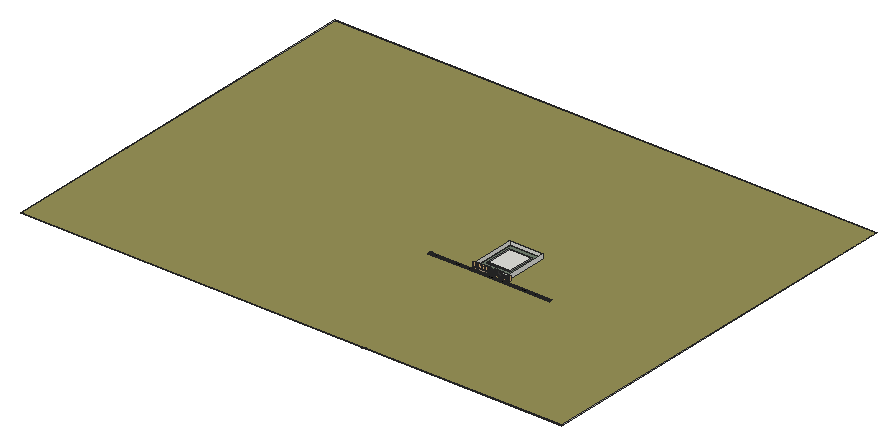
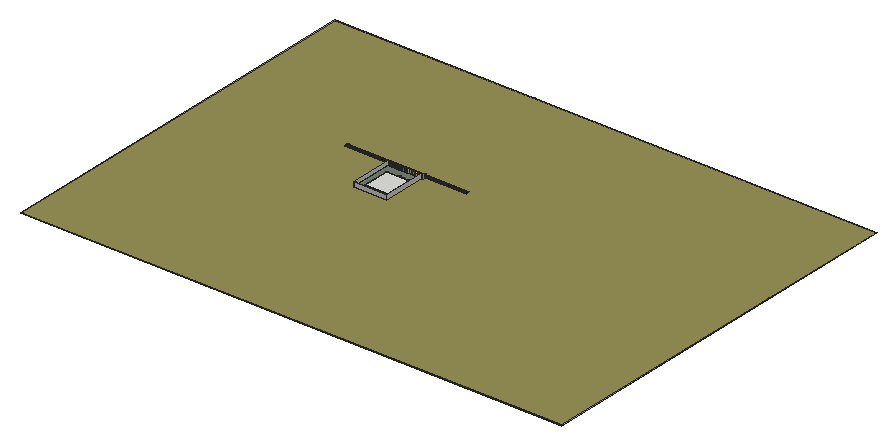
# SketchUp Ruby script. Lengths in inches.
U = 1.inch
M = Sketchup.active_model
def pt(a) = Geom::Point3d.new(a.map { |v| v * U })
def face(e, loops, mat)
  f = e.add_face(loops[0].map { |a| pt(a) })
  loops[1..].each { |l| e.add_face(l.map { |a| pt(a) }).erase! }
  f.material = f.back_material = mat if mat
  f
end
# faces: each face lists its corners as indices into pts; further lists are holes
def faces(e, pts, list, mat = nil) = list.each { |f| face(e, (f[0].is_a?(Array) ? f : [f]).map { |l| l.map { |i| pts[i] } }, mat) }
# xy, xz, yz: faces in a plane at the given z, y or x. An outline is a flat list of corners, or four numbers for a rectangle; further outlines are holes
def ring(l) = l.size == 4 ? [[l[0], l[1]], [l[2], l[1]], [l[2], l[3]], [l[0], l[3]]] : l.each_slice(2).to_a
def flat(e, list, mat, &to3) = list.each { |f| face(e, (f[0].is_a?(Array) ? f : [f]).map { |l| ring(l).map { |u, v| to3.(u, v) } }, mat) }
def xy(e, z, list, mat = nil) = flat(e, list, mat) { |x, y| [x, y, z] }
def xz(e, y, list, mat = nil) = flat(e, list, mat) { |x, z| [x, y, z] }
def yz(e, x, list, mat = nil) = flat(e, list, mat) { |y, z| [x, y, z] }
def lines(e, pts, list) = list.each { |a, b| e.add_line(pt(pts[a]), pt(pts[b])) }
# prism: a flat outline (further loops are holes) pulled along v
def prism(e, loops, v, mat = nil)
  f = face(e, loops, mat); d = Geom::Vector3d.new(v.map { |x| x * U })
  f.pushpull(f.normal.samedirection?(d) ? d.length : -d.length)
end
def box(e, o, s, mat = nil) = prism(e, [[o, [o[0] + s[0], o[1], o[2]], [o[0] + s[0], o[1] + s[1], o[2]], [o[0], o[1] + s[1], o[2]]]], [0, 0, s[2]], mat)
def at(x, y, z, deg = 0) = Geom::Transformation.translation(pt([x, y, z])) * Geom::Transformation.rotation(ORIGIN, Z_AXIS, deg.degrees)
def axes(o, x, y, z) = Geom::Transformation.new([*x, 0, *y, 0, *z, 0, *pt(o).to_a, 1])
def part(name) = M.definitions.add(name)
# library, detail: a bought-in or finely detailed component or shape, given as its bounding box
def library(name, o, s) = part(name).tap { |d| box(d.entities, o, s) }
def detail(e, o, s) = box(e.add_group.entities, o, s)
def put(e, d, t, mat = nil) = e.add_instance(d, t).tap { |i| i.material = mat if mat }
def group(e, t, mat = nil) = e.add_group.tap { |g| g.transformation = t; g.material = mat if mat }.entities
root = M.entities
M.materials.add("C07_Caramel_Shine").color = [153, 76, 0]
M.materials.add("M03_Pewter_Shine").color = [168, 168, 168]
M.materials.add("M07_Charcoal_Gleam").color = [58, 58, 58]
M.materials.add("M09_Shadow_Night").color = [0, 0, 0]
M.materials.add("Marble_01_1K").color = [230, 221, 211]
M.materials.add("Marble_06_1K").color = [165, 150, 147]
M.materials.add("Metal_06_1K").color = [238, 236, 231]
M.materials.add("Plaster_02_1K").color = [157, 140, 119]
M.materials.add("Plaster_04_1K").color = [115, 129, 112]
M.materials.add("Plaster_06_1K").color = [141, 135, 122]
M.materials.add("Plywood_01_1K").color = [125, 96, 64]
M.materials.add("Soil_04_1K").color = [152, 146, 88]
M.materials.add("Wood_Veneer_15_1K").color = [103, 69, 45]
c1 = part("Group\#38")
box(c1.entities,[0,0,0],[5,1.875,282.41],"Metal_06_1K")
c2 = library("Group\#40",[0,0,0],[80.6875,45.375,2.875])
c3 = library("Group\#39",[0,-3.0625,0],[84,3.0625,102])
c4 = part("Group\#43")
xy(c4.entities,0,[[0,-24,550.875,0]])
xy(c4.entities,12.625,[[3.37,-20.63,547.5,-3.37]],"Soil_04_1K")
xy(c4.entities,18,[[[0,-24,550.875,0],[3.37,-20.63,547.5,-3.37]]])
xz(c4.entities,-24,[[0,0,550.875,18]])
xz(c4.entities,-20.63,[[3.37,12.625,547.5,18]])
xz(c4.entities,-3.37,[[3.37,12.625,547.5,18]])
xz(c4.entities,0,[[0,0,550.875,18]])
yz(c4.entities,0,[[-24,0,0,18]])
yz(c4.entities,3.37,[[-20.63,12.625,-3.37,18]])
yz(c4.entities,547.5,[[-20.63,12.625,-3.37,18]])
yz(c4.entities,550.875,[[-24,0,0,18]])
c5 = library("Lantern 03",[-10.78,-12.92,0],[25.67,25.84,111.375])
c6 = library("Deluxe 6’ Bench",[-36.03,-11.33,0.05],[72.04,26.2,31.51])
c7 = part("Group\#46")
box(c7.entities,[0,0,0],[247.875,18.625,1])
g1 = group(root,at(8950.9375,4405.5625,0))
xy(g1,-21,[[-8950.9375,-4405.5625,5495.8125,6096.125]])
xy(g1,-18,[[-8950.9375,-4405.5625,5495.8125,6096.125]],"Soil_04_1K")
xy(g1,0,[[-38.61,-269.5,224.375,-263.5],[224.375,-269.5,250.9375,-263.5],[250.9375,-269.5,775.25,-256.625]])
xy(g1,0,[[-103.0625,-263.5,250.9375,-263.5,250.9375,-256.625,769.25,-256.625,769.25,879.875,-103.0625,879.875]],"Plaster_04_1K")
xy(g1,20.78,[[-92.4,-269.5,-59.27,-268.5]],"C07_Caramel_Shine")
xy(g1,22.41,[[-92.4,-269.5,-59.27,-268.5]],"C07_Caramel_Shine")
xy(g1,29.87,[[-92.4,-269.5,-59.27,-268.5]],"C07_Caramel_Shine")
xy(g1,31.49,[[-92.4,-269.5,-59.27,-268.5]],"C07_Caramel_Shine")
xy(g1,38.95,[[-92.4,-269.5,-59.27,-268.5]],"C07_Caramel_Shine")
xy(g1,40.58,[[-92.4,-269.5,-59.27,-268.5]],"C07_Caramel_Shine")
xy(g1,48.03,[[-92.4,-269.5,-59.27,-268.5]],"C07_Caramel_Shine")
xy(g1,49.66,[[-92.4,-269.5,-59.27,-268.5]],"C07_Caramel_Shine")
xy(g1,57.12,[[-92.4,-269.5,-59.27,-268.5]],"C07_Caramel_Shine")
xy(g1,58.74,[[-92.4,-269.5,-59.27,-268.5]],"C07_Caramel_Shine")
xy(g1,66.2,[[-92.4,-269.5,-59.27,-268.5]],"C07_Caramel_Shine")
xy(g1,67.83,[[-92.4,-269.5,-59.27,-268.5]],"C07_Caramel_Shine")
xy(g1,75.28,[[-92.4,-269.5,-59.27,-268.5]],"C07_Caramel_Shine")
xy(g1,76.91,[[-92.4,-269.5,-59.27,-268.5]],"C07_Caramel_Shine")
xy(g1,96,[[-113.0625,-263.5,-103.0625,-263.5,-103.0625,879.875,769.25,879.875,769.25,-256.625,775.25,-256.625,775.25,885.875,-113.0625,885.875]])
xy(g1,103.5,[[-113.0625,-269.5,-38.61,-263.5]])
xz(g1,-4405.5625,[[-8950.9375,-21,224.375,-18],[224.375,-21,5495.8125,-18]])
xz(g1,-269.5,[[-38.61,-18,224.375,0],[[-113.0625,0,-38.61,103.5],[-92.4,14.67,-59.27,82.01]]])
xz(g1,-269.5,[[-92.4,14.67,-59.27,20.78],[-92.4,22.41,-59.27,29.87],[-92.4,31.49,-59.27,38.95],[-92.4,40.58,-59.27,48.03],[-92.4,49.66,-59.27,57.12],
  [-92.4,58.74,-59.27,66.2],[-92.4,67.83,-59.27,75.28],[-92.4,76.91,-59.27,82.01]],"Wood_Veneer_15_1K")
xz(g1,-268.5,[[-92.4,20.78,-59.27,22.41],[-92.4,29.87,-59.27,31.49],[-92.4,38.95,-59.27,40.58],[-92.4,48.03,-59.27,49.66],[-92.4,57.12,-59.27,58.74],
  [-92.4,66.2,-59.27,67.83],[-92.4,75.28,-59.27,76.91]],"C07_Caramel_Shine")
xz(g1,-263.5,[[-103.0625,0,-38.61,103.5],[-113.0625,96,-103.0625,103.5]])
xz(g1,-256.625,[[769.25,0,775.25,96]])
xz(g1,879.875,[[-103.0625,0,769.25,96]])
xz(g1,885.875,[[-113.0625,-18,775.25,96]])
xz(g1,6096.125,[[-8950.9375,-21,5495.8125,-18]])
yz(g1,-8950.9375,[[-4405.5625,-21,-837.25,-18],[-837.25,-21,6096.125,-18]])
yz(g1,-113.0625,[[-269.5,-18,-269.5,103.5,-263.5,103.5,-263.5,96,885.875,96,885.875,-18]])
yz(g1,-103.0625,[[-263.5,0,879.875,96]])
yz(g1,-92.4,[[-269.5,20.78,-268.5,22.41],[-269.5,29.87,-268.5,31.49],[-269.5,38.95,-268.5,40.58],[-269.5,48.03,-268.5,49.66],[-269.5,57.12,-268.5,58.74],
  [-269.5,66.2,-268.5,67.83],[-269.5,75.28,-268.5,76.91]],"C07_Caramel_Shine")
yz(g1,-59.27,[[-269.5,20.78,-268.5,22.41],[-269.5,29.87,-268.5,31.49],[-269.5,38.95,-268.5,40.58],[-269.5,48.03,-268.5,49.66],[-269.5,57.12,-268.5,58.74],
  [-269.5,66.2,-268.5,67.83],[-269.5,75.28,-268.5,76.91]],"C07_Caramel_Shine")
yz(g1,-38.61,[[-269.5,0,-263.5,103.5]])
yz(g1,769.25,[[-256.625,0,879.875,96]])
yz(g1,775.25,[[-269.5,-18,885.875,-18,885.875,96,-256.625,96,-256.625,0,-269.5,0]])
yz(g1,5495.8125,[[-4405.5625,-21,6096.125,-18]])
g2 = group(g1,at(250.9375,-269.5,0))
xy(g2,0,[[-2.57,0,-2.57,8.6875,143.56,8.6875,143.56,12.875,340.42,12.875,340.42,0],[465.96,0,524.3125,12.875]])
xy(g2,24,[[-2.57,0,143.56,3.25]],"M07_Charcoal_Gleam")
xy(g2,33.26,[[183.55,0,216.43,12.875]])
xy(g2,71.1875,[[183.55,0,216.43,12.875],[340.42,0,465.96,12.875]])
xy(g2,90.75,[[-2.57,3.25,143.56,8.6875]],"Plaster_06_1K")
xy(g2,103.5,[[340.42,0,524.3125,12.875]])
xy(g2,103.5,[[143.56,0,183.55,12.875],[216.43,0,340.42,12.875]],"M07_Charcoal_Gleam")
xy(g2,107.875,[[183.55,0,216.43,12.875]])
xz(g2,0,[[465.96,0,524.3125,0,524.3125,103.5,340.42,103.5,340.42,95.1875,248.6,95.1875,248.6,71.1875,465.96,71.1875],[183.55,71.1875,216.43,107.875]])
xz(g2,0,[[-2.57,0,340.42,0,340.42,71.1875,248.6,71.1875,248.6,95.1875,340.42,95.1875,340.42,103.5,216.43,103.5,216.43,33.26,183.55,33.26,183.55,103.5,143.56,103.5,143.56,24,-2.57,24]],"M07_Charcoal_Gleam")
xz(g2,3.25,[[-2.57,24,143.56,90.75]],"Plaster_06_1K")
xz(g2,8.6875,[[-2.57,0,143.56,90.75]],"Plaster_06_1K")
xz(g2,12.875,[[465.96,0,465.96,71.1875,340.42,71.1875,340.42,103.5,518.3125,103.5,518.3125,0],[518.3125,0,524.3125,103.5]])
xz(g2,12.875,[[[143.56,0,143.56,103.5,183.55,103.5,183.55,107.875,216.43,107.875,216.43,103.5,340.42,103.5,340.42,0],[183.55,33.26,216.43,71.1875]]],"M07_Charcoal_Gleam")
yz(g2,-2.57,[[0,0,0,24,3.25,24,3.25,90.75,6,90.75,6,0],[6,0,8.6875,90.75]])
yz(g2,143.56,[[8.6875,0,8.6875,90.75,3.25,90.75,3.25,24,0,24,0,103.5,12.875,103.5,12.875,0]],"M07_Charcoal_Gleam")
yz(g2,183.55,[[0,33.26,12.875,71.1875],[0,103.5,12.875,107.875]])
yz(g2,216.43,[[0,33.26,12.875,71.1875],[0,103.5,12.875,107.875]])
yz(g2,340.42,[[0,0,12.875,71.1875]],"M07_Charcoal_Gleam")
yz(g2,465.96,[[0,0,12.875,71.1875]])
yz(g2,524.3125,[[0,0,12.875,103.5]])
put(g2,c1,axes([465.96,8.52,66.9],[0,-1,0],[0,0,1],[-1,0,0]))
put(g2,c1,axes([465.96,8.52,57.86],[0,-1,0],[0,0,1],[-1,0,0]))
put(g2,c1,axes([465.96,8.52,48.82],[0,-1,0],[0,0,1],[-1,0,0]))
put(g2,c1,axes([465.96,8.52,39.79],[0,-1,0],[0,0,1],[-1,0,0]))
put(g2,c1,axes([465.96,8.52,30.75],[0,-1,0],[0,0,1],[-1,0,0]))
put(g2,c1,axes([465.96,8.52,21.72],[0,-1,0],[0,0,1],[-1,0,0]))
put(g2,c1,axes([465.96,8.52,12.68],[0,-1,0],[0,0,1],[-1,0,0]))
put(g2,c1,axes([465.96,8.52,3.65],[0,-1,0],[0,0,1],[-1,0,0]))
put(g2,c2,axes([27.93,3.25,33.82],[1,0,0],[0,0,1],[0,-1,0]))
put(g1,c3,axes([-38.61,-266.5,0],[1.03996,0,0],[0,1,0],[0,0,0.9408]))
put(g1,c3,axes([49.66,-266.5,0],[1.03996,0,0],[0,1,0],[0,0,0.9408]))
put(g1,c3,axes([137.02,-266.5,0],[1.03996,0,0],[0,1,0],[0,0,0.9408]))
g3 = group(g1,at(-113.0625,-269.5,-18))
xy(g3,0,[[0,-24,74.46,0]])
xy(g3,12.625,[[3.37,-20.63,71.08,-3.37]],"Soil_04_1K")
xy(g3,18,[[[0,-24,74.46,0],[3.37,-20.63,71.08,-3.37]]])
xz(g3,-24,[[0,0,74.46,18]])
xz(g3,-20.63,[[3.37,12.625,71.08,18]])
xz(g3,-3.37,[[3.37,12.625,71.08,18]])
xz(g3,0,[[0,0,74.46,18]])
yz(g3,0,[[-24,0,0,18]])
yz(g3,3.37,[[-20.63,12.625,-3.37,18]])
yz(g3,71.08,[[-20.63,12.625,-3.37,18]])
yz(g3,74.46,[[-24,0,0,18]])
put(g1,c4,axes([224.375,-269.5,-18],[0.4,0,0],[0,1,0],[0,0,1]))
put(g1,c4,axes([444.72,-269.5,-18],[0.4,0,0],[0,1,0],[0,0,1]))
put(g1,c4,axes([665.07,-269.5,-18],[0.2,0,0],[0,1,0],[0,0,1]))
put(root,c5,at(8801.1,4116.48,-18))
put(root,c5,at(9769.7,4127.8,-18))
g4 = group(root,at(8912.33,4041.91,-18))
xy(g4,0,[[0,0,262.98,94.16]],"Plaster_02_1K")
yz(g4,0,[[0,0,70.16,0,70.16,13.41]],"Plaster_02_1K")
yz(g4,262.98,[[0,0,70.04,13.39,70.04,0]],"Plaster_02_1K")
p = [[262.98,94.16,18],[262.98,70.04,13.39],[262.98,0,0],[0,0,0],[0,70.16,13.41],[0,94.16,18]]
faces(g4,p,[[0,1,2,3,4,5]],"Plaster_02_1K")
g5 = group(root,at(7707.8125,3957.91,-18))
prism(g5,[[[3255.3125,84,0],[3255.3125,0,0],[1204.52,0,0],[0,0,0],[0,84,0],[1204.52,84,0]]],[0,0,1],"M09_Shadow_Night")
put(root,c6,at(8864.21,4064.76,-18),"Plywood_01_1K")
put(root,c6,at(9632.09,4062.93,-18),"Plywood_01_1K")
put(root,c6,at(9421.9,4064.97,-18),"Plywood_01_1K")
put(root,c7,at(7764.95,3998.1,-17))
put(root,c7,at(8058.52,3998.1,-17))
put(root,c7,at(8352.09,3998.1,-17))
put(root,c7,at(8645.65,3998.1,-17))
put(root,c7,at(8939.22,3998.1,-17))
put(root,c7,at(9232.79,3998.1,-17))
put(root,c7,at(9526.36,3998.1,-17))
put(root,c7,at(9819.93,3998.1,-17))
put(root,c7,at(10113.5,3998.1,-17))
put(root,c7,at(10407.07,3998.1,-17))
put(root,c7,at(10700.64,3998.1,-17))
g6 = group(root,at(8950.9375,4405.5625,0))
xy(g6,0,[[281.36,-20.91,-0.06,-20,0,0,281.43,-0.91],[0,0,600,720]])
xy(g6,6,[[281.36,-20.91,281.4,-10.91,-0.03,-10,-0.06,-20]],"Marble_06_1K")
xy(g6,12,[[281.4,-10.91,281.43,-0.91,0,0,-0.03,-10]],"Marble_06_1K")
xy(g6,18,[[0,0,600,720]])
xz(g6,0,[[0,0,600,18]],"M03_Pewter_Shine")
xz(g6,720,[[0,0,600,18]],"M03_Pewter_Shine")
yz(g6,0,[[0,0,720,18]],"M03_Pewter_Shine")
yz(g6,600,[[0,0,720,18]],"M03_Pewter_Shine")
p = [[281.36,-20.91,0],[281.36,-20.91,6],[-0.06,-20,6],[-0.06,-20,0],[281.43,-0.91,0],[281.43,-0.91,12],
  [281.4,-10.91,12],[281.4,-10.91,6],[0,0,12],[0,0,0],[-0.03,-10,6],[-0.03,-10,12],
  [281.43,-0.91,18],[0,0,18],[12,0,18],[281.43,-0.91,24],[12,0,24]]
faces(g6,p,[[0,1,2,3],[6,11,10,7],[12,13,8,5],[14,12,15,16]],"Marble_06_1K")
faces(g6,p,[[0,4,5,6,7,1],[8,9,3,2,10,11]],"Marble_01_1K")
g7 = group(root,at(9175.3125,4136.0625,0))
box(g7,[0,0,0],[24,13.68,107.875])
